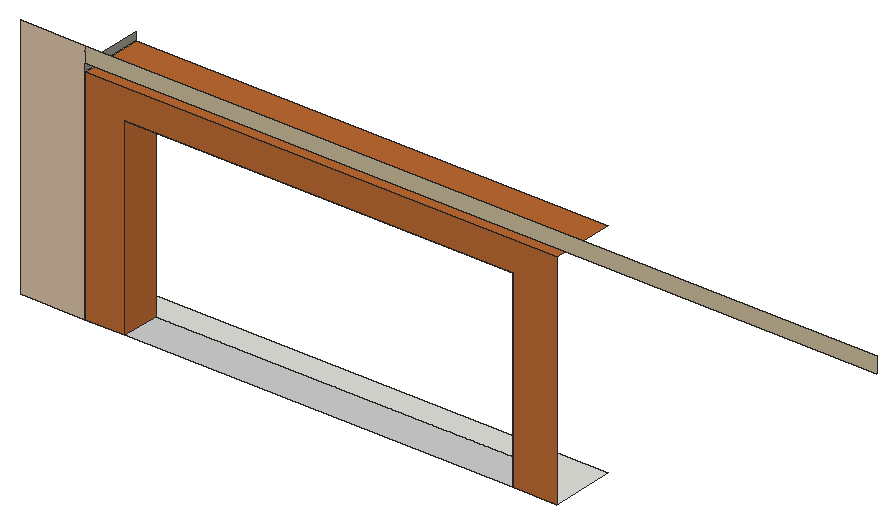
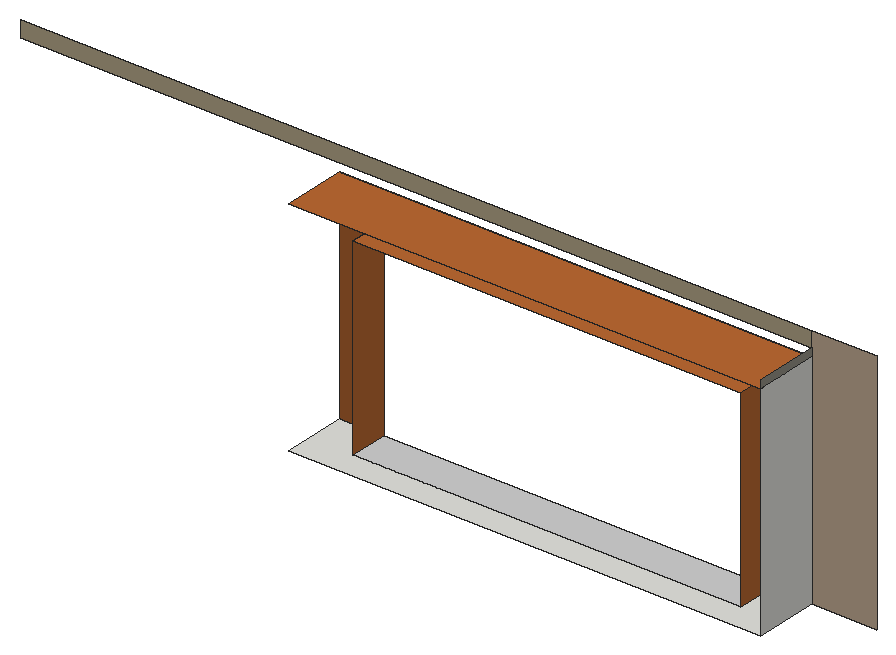
# SketchUp Ruby script. Lengths in inches.
U = 1.inch
M = Sketchup.active_model
def pt(a) = Geom::Point3d.new(a.map { |v| v * U })
def face(e, loops, mat)
  f = e.add_face(loops[0].map { |a| pt(a) })
  loops[1..].each { |l| e.add_face(l.map { |a| pt(a) }).erase! }
  f.material = f.back_material = mat if mat
  f
end
# faces: each face lists its corners as indices into pts; further lists are holes
def faces(e, pts, list, mat = nil) = list.each { |f| face(e, (f[0].is_a?(Array) ? f : [f]).map { |l| l.map { |i| pts[i] } }, mat) }
# xy, xz, yz: faces in a plane at the given z, y or x. An outline is a flat list of corners, or four numbers for a rectangle; further outlines are holes
def ring(l) = l.size == 4 ? [[l[0], l[1]], [l[2], l[1]], [l[2], l[3]], [l[0], l[3]]] : l.each_slice(2).to_a
def flat(e, list, mat, &to3) = list.each { |f| face(e, (f[0].is_a?(Array) ? f : [f]).map { |l| ring(l).map { |u, v| to3.(u, v) } }, mat) }
def xy(e, z, list, mat = nil) = flat(e, list, mat) { |x, y| [x, y, z] }
def xz(e, y, list, mat = nil) = flat(e, list, mat) { |x, z| [x, y, z] }
def yz(e, x, list, mat = nil) = flat(e, list, mat) { |y, z| [x, y, z] }
def lines(e, pts, list) = list.each { |a, b| e.add_line(pt(pts[a]), pt(pts[b])) }
# prism: a flat outline (further loops are holes) pulled along v
def prism(e, loops, v, mat = nil)
  f = face(e, loops, mat); d = Geom::Vector3d.new(v.map { |x| x * U })
  f.pushpull(f.normal.samedirection?(d) ? d.length : -d.length)
end
def box(e, o, s, mat = nil) = prism(e, [[o, [o[0] + s[0], o[1], o[2]], [o[0] + s[0], o[1] + s[1], o[2]], [o[0], o[1] + s[1], o[2]]]], [0, 0, s[2]], mat)
def at(x, y, z, deg = 0) = Geom::Transformation.translation(pt([x, y, z])) * Geom::Transformation.rotation(ORIGIN, Z_AXIS, deg.degrees)
def axes(o, x, y, z) = Geom::Transformation.new([*x, 0, *y, 0, *z, 0, *pt(o).to_a, 1])
def part(name) = M.definitions.add(name)
# library, detail: a bought-in or finely detailed component or shape, given as its bounding box
def library(name, o, s) = part(name).tap { |d| box(d.entities, o, s) }
def detail(e, o, s) = box(e.add_group.entities, o, s)
def put(e, d, t, mat = nil) = e.add_instance(d, t).tap { |i| i.material = mat if mat }
def group(e, t, mat = nil) = e.add_group.tap { |g| g.transformation = t; g.material = mat if mat }.entities
root = M.entities
M.materials.add("[Carrera Marble]").color = [207, 207, 207]
M.materials.add("[Formica Graystone]").color = [149, 146, 135]
M.materials.add("[Formica Laminate Light]").color = [213, 189, 164]
M.materials.add("[Quartz Light Brown]").color = [199, 184, 152]
M.materials.add("[Wood Cherry Original]").color = [186, 105, 51]
xy(root,0,[[24.17,184.11,24.17,208.28,201.37,208.28,201.37,184.11,185.03,184.11,185.03,198.55,39.34,198.55,39.34,184.11]])
xy(root,0,[[39.34,184.11,185.03,198.55]],"[Carrera Marble]")
xy(root,72.25,[[39.34,184.11,185.03,198.55]],"[Wood Cherry Original]")
xy(root,83.1875,[[24.17,184.11,201.37,208.28]],"[Wood Cherry Original]")
xz(root,184.11,[[0,0,24.17,92.125]],"[Formica Laminate Light]")
xz(root,184.11,[[24.17,86.16,321.5,92.125]],"[Quartz Light Brown]")
xz(root,184.11,[[24.17,0,39.34,0,39.34,72.25,185.03,72.25,185.03,0,201.37,0,201.37,83.1875,24.17,83.1875]],"[Wood Cherry Original]")
yz(root,24.17,[[184.11,0,208.28,83.1875]])
yz(root,24.17,[[184.11,83.1875,208.28,86.16]],"[Formica Graystone]")
yz(root,39.34,[[184.11,0,198.55,72.25]],"[Wood Cherry Original]")
yz(root,185.03,[[184.11,0,198.55,72.25]],"[Wood Cherry Original]")
